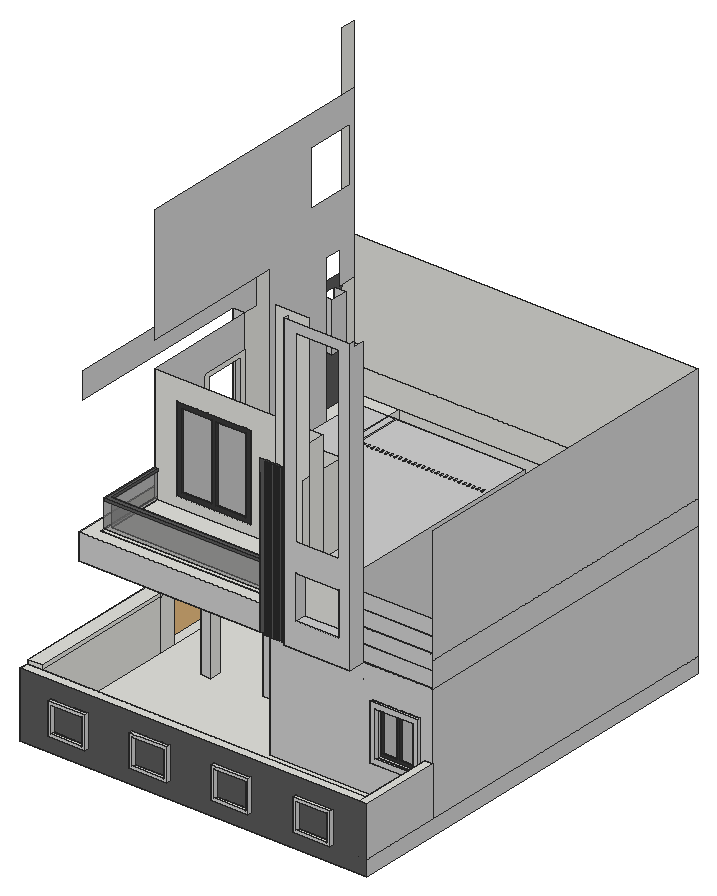
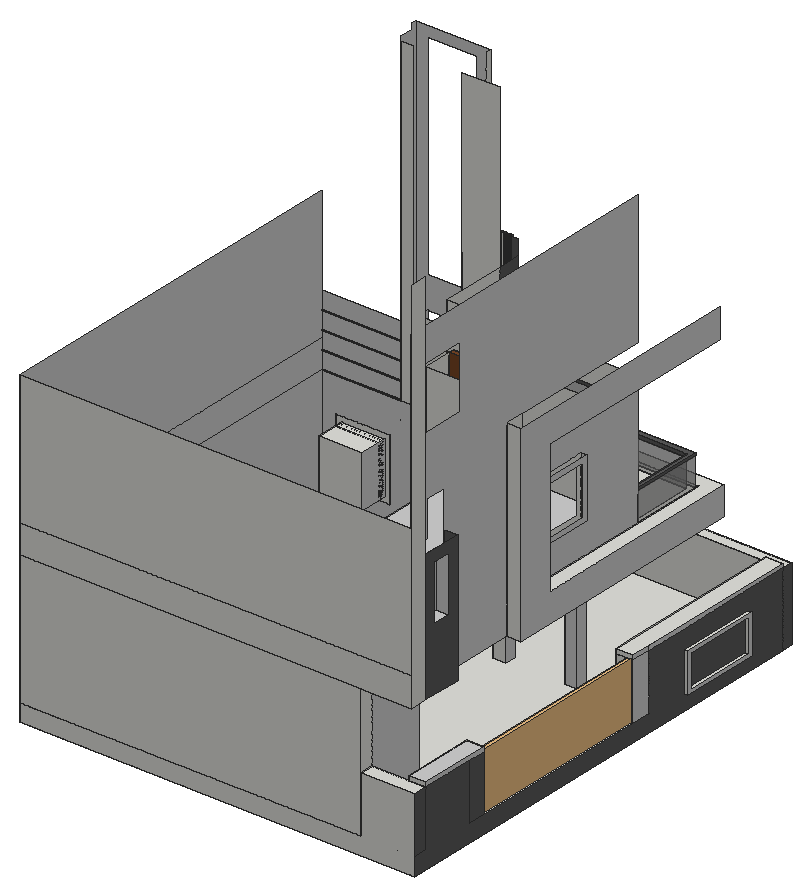
# SketchUp Ruby script. Lengths in inches.
U = 1.inch
M = Sketchup.active_model
def pt(a) = Geom::Point3d.new(a.map { |v| v * U })
def face(e, loops, mat)
  f = e.add_face(loops[0].map { |a| pt(a) })
  loops[1..].each { |l| e.add_face(l.map { |a| pt(a) }).erase! }
  f.material = f.back_material = mat if mat
  f
end
# faces: each face lists its corners as indices into pts; further lists are holes
def faces(e, pts, list, mat = nil) = list.each { |f| face(e, (f[0].is_a?(Array) ? f : [f]).map { |l| l.map { |i| pts[i] } }, mat) }
# xy, xz, yz: faces in a plane at the given z, y or x. An outline is a flat list of corners, or four numbers for a rectangle; further outlines are holes
def ring(l) = l.size == 4 ? [[l[0], l[1]], [l[2], l[1]], [l[2], l[3]], [l[0], l[3]]] : l.each_slice(2).to_a
def flat(e, list, mat, &to3) = list.each { |f| face(e, (f[0].is_a?(Array) ? f : [f]).map { |l| ring(l).map { |u, v| to3.(u, v) } }, mat) }
def xy(e, z, list, mat = nil) = flat(e, list, mat) { |x, y| [x, y, z] }
def xz(e, y, list, mat = nil) = flat(e, list, mat) { |x, z| [x, y, z] }
def yz(e, x, list, mat = nil) = flat(e, list, mat) { |y, z| [x, y, z] }
def lines(e, pts, list) = list.each { |a, b| e.add_line(pt(pts[a]), pt(pts[b])) }
# prism: a flat outline (further loops are holes) pulled along v
def prism(e, loops, v, mat = nil)
  f = face(e, loops, mat); d = Geom::Vector3d.new(v.map { |x| x * U })
  f.pushpull(f.normal.samedirection?(d) ? d.length : -d.length)
end
def box(e, o, s, mat = nil) = prism(e, [[o, [o[0] + s[0], o[1], o[2]], [o[0] + s[0], o[1] + s[1], o[2]], [o[0], o[1] + s[1], o[2]]]], [0, 0, s[2]], mat)
def at(x, y, z, deg = 0) = Geom::Transformation.translation(pt([x, y, z])) * Geom::Transformation.rotation(ORIGIN, Z_AXIS, deg.degrees)
def axes(o, x, y, z) = Geom::Transformation.new([*x, 0, *y, 0, *z, 0, *pt(o).to_a, 1])
def part(name) = M.definitions.add(name)
# library, detail: a bought-in or finely detailed component or shape, given as its bounding box
def library(name, o, s) = part(name).tap { |d| box(d.entities, o, s) }
def detail(e, o, s) = box(e.add_group.entities, o, s)
def put(e, d, t, mat = nil) = e.add_instance(d, t).tap { |i| i.material = mat if mat }
def group(e, t, mat = nil) = e.add_group.tap { |g| g.transformation = t; g.material = mat if mat }.entities
root = M.entities
M.materials.add("Generic").color = [90, 90, 90]
M.materials.add("Generic\#1").color = [208, 208, 208]
M.materials.add("[Color M07]").color = [58, 58, 58]
M.materials.add("[Mirror 01]").color = [185, 185, 185]
M.materials.add("[Translucent Glass Gray]").color = [128, 128, 128]
M.materials["[Translucent Glass Gray]"].alpha = 0.5
M.materials.add("[Wood Bamboo]").color = [177, 105, 43]
M.materials.add("[Wood Veneer 01]").color = [120, 70, 37]
c1 = library("Group\#6",[0,0,0],[5.12,237.75,72])
c2 = part("Group\#5")
xy(c2.entities,225.125,[[0,0,3,3.25]])
xz(c2.entities,0,[[0,0,3,225.125]])
yz(c2.entities,0,[[0,0,3.25,225.125]])
yz(c2.entities,3,[[0,0,3.25,225.125]])
c3 = part("Group\#8")
xy(c3.entities,0,[[0,0,56.875,6.5]],"[Wood Veneer 01]")
xy(c3.entities,4.88,[[4.88,0,51.99,3.5]],"[Wood Veneer 01]")
xy(c3.entities,109.93,[[4.88,0,51.99,3.5]],"[Wood Veneer 01]")
xy(c3.entities,114.8125,[[0,0,56.875,6.5]],"[Wood Veneer 01]")
xz(c3.entities,0,[[[0,0,56.875,114.8125],[4.88,4.88,51.99,109.93]]],"[Wood Veneer 01]")
xz(c3.entities,0.5,[[8.38,56.46,8.6,56.49,8.8,56.57,8.97,56.7,9.1,56.88,9.1875,57.08,9.22,57.3,9.1875,57.51,9.1,57.71,8.97,57.89,8.8,58.02,8.6,58.1,8.38,58.13,8.16,58.1,7.96,58.02,7.79,57.89,7.66,57.71,7.57,57.51,7.54,57.3,7.57,57.08,7.66,56.88,7.79,56.7,7.96,56.57,8.16,56.49]],"[Wood Veneer 01]")
xz(c3.entities,3.5,[[8.38,56.46,8.16,56.49,7.96,56.57,7.79,56.7,7.66,56.88,7.57,57.08,7.54,57.3,7.57,57.51,7.66,57.71,7.79,57.89,7.96,58.02,8.16,58.1,8.38,58.13,8.6,58.1,8.8,58.02,8.97,57.89,9.1,57.71,9.1875,57.51,9.22,57.3,9.1875,57.08,9.1,56.88,8.97,56.7,8.8,56.57,8.6,56.49]])
xz(c3.entities,3.5,[[[4.88,4.88,51.99,109.93],[8.38,56.46,8.16,56.49,7.96,56.57,7.79,56.7,7.66,56.88,7.57,57.08,7.54,57.3,7.57,57.51,7.66,57.71,7.79,57.89,7.96,58.02,8.16,58.1,8.38,58.13,8.6,58.1,8.8,58.02,8.97,57.89,9.1,57.71,9.1875,57.51,9.22,57.3,9.1875,57.08,9.1,56.88,8.97,56.7,8.8,56.57,8.6,56.49]]],"[Wood Bamboo]")
xz(c3.entities,6.5,[[0,0,56.875,114.8125]],"[Wood Veneer 01]")
yz(c3.entities,0,[[0,0,6.5,114.8125]],"[Wood Veneer 01]")
yz(c3.entities,4.88,[[0,4.88,3.5,109.93]],"[Wood Veneer 01]")
yz(c3.entities,51.99,[[0,4.88,3.5,109.93]],"[Wood Veneer 01]")
yz(c3.entities,56.875,[[0,0,6.5,114.8125]],"[Wood Veneer 01]")
p = [[7.96,3.5,56.57],[8.16,3.5,56.49],[8.16,0.5,56.49],[7.96,0.5,56.57],[8.38,3.5,56.46],[8.38,0.5,56.46],
  [8.6,3.5,56.49],[8.6,0.5,56.49],[8.8,3.5,56.57],[8.8,0.5,56.57],[7.79,3.5,56.7],[7.79,0.5,56.7],
  [8.97,3.5,56.7],[8.97,0.5,56.7],[7.66,3.5,56.88],[7.66,0.5,56.88],[9.1,3.5,56.88],[9.1,0.5,56.88],
  [7.57,3.5,57.08],[7.57,0.5,57.08],[9.1875,3.5,57.08],[9.1875,0.5,57.08],[7.54,3.5,57.3],[7.54,0.5,57.3],
  [9.22,3.5,57.3],[9.22,0.5,57.3],[7.57,3.5,57.51],[7.57,0.5,57.51],[9.1875,3.5,57.51],[9.1875,0.5,57.51],
  [7.66,3.5,57.71],[7.66,0.5,57.71],[9.1,3.5,57.71],[9.1,0.5,57.71],[7.79,3.5,57.89],[7.79,0.5,57.89],
  [8.97,3.5,57.89],[8.97,0.5,57.89],[7.96,3.5,58.02],[7.96,0.5,58.02],[8.8,3.5,58.02],[8.8,0.5,58.02],
  [8.16,3.5,58.1],[8.16,0.5,58.1],[8.6,3.5,58.1],[8.6,0.5,58.1],[8.38,3.5,58.13],[8.38,0.5,58.13],
  [8.38,3.5,57.3],[8.38,0.5,57.3]]
faces(c3.entities,p,[[0,1,2,3],[1,4,5,2],[4,6,7,5],[6,8,9,7],[10,0,3,11],[8,12,13,9],[14,10,11,15],[12,16,17,13],
  [18,14,15,19],[16,20,21,17],[22,18,19,23],[20,24,25,21],[26,22,23,27],[24,28,29,25],[30,26,27,31],[28,32,33,29],
  [34,30,31,35],[32,36,37,33],[38,34,35,39],[36,40,41,37],[42,38,39,43],[40,44,45,41],[46,42,43,47],[44,46,47,45]],"[Wood Veneer 01]")
lines(c3.entities,p,[[48,49]])
c4 = part("Group\#7")
xy(c4.entities,0,[[0,0,106.25,6]],"[Color M07]")
xy(c4.entities,6.42,[[6.42,0,49.92,3],[56.33,0,99.83,3]],"[Color M07]")
xy(c4.entities,116.15,[[6.42,0,49.92,3],[56.33,0,99.83,3]],"[Color M07]")
xy(c4.entities,122.5625,[[0,0,106.25,6]],"[Color M07]")
xz(c4.entities,0,[[[0,0,106.25,122.5625],[56.33,6.42,99.83,116.15],[6.42,6.42,49.92,116.15]]],"[Color M07]")
xz(c4.entities,3,[[6.42,6.42,49.92,116.15],[56.33,6.42,99.83,116.15]],"[Mirror 01]")
xz(c4.entities,6,[[0,0,106.25,122.5625]],"[Mirror 01]")
yz(c4.entities,0,[[0,0,6,122.5625]],"[Color M07]")
yz(c4.entities,6.42,[[0,6.42,3,116.15]],"[Color M07]")
yz(c4.entities,49.92,[[0,6.42,3,116.15]],"[Color M07]")
yz(c4.entities,56.33,[[0,6.42,3,116.15]],"[Color M07]")
yz(c4.entities,99.83,[[0,6.42,3,116.15]],"[Color M07]")
yz(c4.entities,106.25,[[0,0,6,122.5625]],"[Color M07]")
xy(root,-21.6875,[[5.4375,5.4375,507.1875,19],[5.4375,19,27.1875,605.125],[27.1875,19,507.1875,605.125]])
xy(root,-1.26,[[0,75.49,5.4375,176.95]],"Generic\#1")
xy(root,0,[[[27.1875,19,495.5625,19,495.5625,125.125,271.1875,125.125,271.1875,512.5,251.64,512.5,251.64,524.5,199.78,524.5,199.78,512.5,73.6875,512.5,73.6875,587,27.1875,587],[180.62,226.81,197.18,241.25],[93.57,221.98,108.82,237.23]],[495.5625,19,507.1875,125.125],[271.1875,125.125,507.1875,125.125,507.1875,605.125,73.6875,605.125,73.6875,587,271.1875,587],[5.4375,233.125,27.1875,257.3125],[5.4375,257.3125,27.1875,495.0625],
  [5.4375,495.0625,27.1875,519.25],[85,524.5,271.1875,587]])
xy(root,0,[[73.6875,512.5,85,587],[85,512.5,199.78,524.5],[251.64,512.5,271.1875,524.5]],"Generic\#1")
xy(root,1.89,[[404.83,0,458.61,5.4375]])
xy(root,1.89,[[49.9,0,103.67,5.4375],[168.21,0,221.98,5.4375],[286.52,0,340.3,5.4375]],"Generic\#1")
xy(root,2.75,[[0,79.5,5.4375,172.9375]])
xy(root,5.91,[[53.91,0,99.66,5.4375],[290.53,0,336.28,5.4375],[408.85,0,454.6,5.4375]])
xy(root,5.91,[[172.22,0,217.97,5.4375]],"Generic\#1")
xy(root,44.09,[[408.85,0,454.6,5.4375]])
xy(root,44.09,[[53.91,0,99.66,5.4375],[172.22,0,217.97,5.4375],[290.53,0,336.28,5.4375]],"Generic\#1")
xy(root,44.88,[[0,79.5,5.4375,172.9375]])
xy(root,45.03,[[420.53,120.5625,489.125,125.125]])
xy(root,48.11,[[404.83,0,458.61,5.4375]])
xy(root,48.11,[[49.9,0,103.67,5.4375],[168.21,0,221.98,5.4375],[286.52,0,340.3,5.4375]],"Generic\#1")
xy(root,48.89,[[0,75.49,5.4375,176.95]])
xy(root,51.86,[[427.36,120.5625,482.3,125.125],[427.36,125.125,482.3,160.875]],"Generic\#1")
xy(root,72,[[5.4375,5.4375,495.5625,19],[495.5625,5.4375,507.1875,125.125],[5.4375,19,27.1875,233.125],[5.4375,233.125,27.1875,257.3125],[5.4375,495.0625,27.1875,519.25],
  [5.4375,519.25,27.1875,587],[5.4375,587,73.6875,605.125]])
xy(root,77.5,[[5.4375,19,27.1875,257.3125]])
xy(root,77.5,[[5.4375,495.0625,27.1875,587]],"Generic\#1")
xy(root,89.9375,[[199.78,512.5,251.64,524.5]],"Generic\#1")
xy(root,117.55,[[427.36,120.5625,482.3,125.125],[427.36,125.125,482.3,160.875]])
xy(root,124.375,[[420.53,120.5625,489.125,125.125]],"Generic\#1")
xy(root,131.75,[[[85,512.5,271.1875,512.5,271.1875,516.95,270.34,516.95,270.34,521.26,271.1875,521.26,271.1875,524.5,85,524.5],[263.71,516.95,265.46,521.26],[257.09,516.95,258.84,521.26],[250.46,516.95,252.21,521.26],[243.84,516.95,245.59,521.26],[237.21,516.95,238.96,521.26],[230.59,516.95,232.34,521.26],[223.96,516.95,225.71,521.26],[217.34,516.95,219.09,521.26],[204.09,516.95,205.84,521.26],[197.46,516.95,199.21,521.26],[190.84,516.95,192.59,521.26],[184.21,516.95,185.96,521.26],[177.59,516.95,179.34,521.26],[170.96,516.95,172.71,521.26],[164.34,516.95,166.09,521.26],[157.71,516.95,159.46,521.26],[151.09,516.95,152.84,521.26],[144.46,516.95,146.21,521.26],[137.84,516.95,139.59,521.26],[131.21,516.95,132.96,521.26],[124.59,516.95,126.34,521.26],[117.96,516.95,119.71,521.26],[111.34,516.95,113.09,521.26],[104.71,516.95,106.46,521.26],[98.09,516.95,99.84,521.26],[91.46,516.95,93.21,521.26],[210.71,516.95,212.46,521.26]],[91.46,516.95,93.21,521.26],[98.09,516.95,99.84,521.26],[104.71,516.95,106.46,521.26],[111.34,516.95,113.09,521.26],
  [117.96,516.95,119.71,521.26],[124.59,516.95,126.34,521.26],[131.21,516.95,132.96,521.26],[137.84,516.95,139.59,521.26],[144.46,516.95,146.21,521.26],
  [151.09,516.95,152.84,521.26],[157.71,516.95,159.46,521.26],[164.34,516.95,166.09,521.26],[170.96,516.95,172.71,521.26],[177.59,516.95,179.34,521.26],
  [184.21,516.95,185.96,521.26],[190.84,516.95,192.59,521.26],[197.46,516.95,199.21,521.26],[204.09,516.95,205.84,521.26],[210.71,516.95,212.46,521.26],
  [217.34,516.95,219.09,521.26],[223.96,516.95,225.71,521.26],[230.59,516.95,232.34,521.26],[237.21,516.95,238.96,521.26],[243.84,516.95,245.59,521.26],
  [250.46,516.95,252.21,521.26],[257.09,516.95,258.84,521.26],[263.71,516.95,265.46,521.26],[270.34,516.95,271.1875,521.26],[271.1875,516.95,272.09,521.26],
  [276.96,516.95,278.71,521.26],[283.59,516.95,285.34,521.26],[290.21,516.95,291.96,521.26],[296.84,516.95,298.59,521.26],[303.46,516.95,305.21,521.26],
  [310.09,516.95,311.84,521.26],[316.71,516.95,318.46,521.26],[323.34,516.95,325.09,521.26],[329.96,516.95,331.71,521.26],[336.59,516.95,338.34,521.26],
  [343.21,516.95,344.96,521.26],[349.84,516.95,351.59,521.26],[356.46,516.95,358.21,521.26],[363.09,516.95,364.84,521.26],[369.71,516.95,371.46,521.26]],"Generic\#1")
xy(root,168,[[311.625,101.1875,328.9375,108.0625],[9.25,531.8125,27.1875,583.375],[9.25,583.375,9.25,605.125,73.6875,605.125,73.6875,587,27.1875,587,27.1875,583.375]])
xy(root,168,[[328.9375,101.1875,328.9375,108.0625,307.5625,108.0625,307.5625,104.8125,304.5625,104.8125,304.5625,108.0625,271.1875,108.0625,271.1875,125.125,406.8125,125.125,406.8125,101.1875],[9.25,108.0625,9.25,430.9,27.1875,430.9,27.1875,125.125,271.1875,125.125,271.1875,108.0625],[[27.1875,125.125,27.1875,587,73.6875,587,73.6875,512.5,85,512.5,85,587,271.1875,587,271.1875,125.125],[180.62,226.81,197.18,241.25],[93.57,221.98,108.82,237.23],[91.46,516.95,93.21,521.26],[98.09,516.95,99.84,521.26],[104.71,516.95,106.46,521.26],[111.34,516.95,113.09,521.26],[117.96,516.95,119.71,521.26],[124.59,516.95,126.34,521.26],[131.21,516.95,132.96,521.26],[137.84,516.95,139.59,521.26],[144.46,516.95,146.21,521.26],[151.09,516.95,152.84,521.26],[157.71,516.95,159.46,521.26],[164.34,516.95,166.09,521.26],[170.96,516.95,172.71,521.26],[263.71,516.95,265.46,521.26],[257.09,516.95,258.84,521.26],[250.46,516.95,252.21,521.26],[243.84,516.95,245.59,521.26],[237.21,516.95,238.96,521.26],[230.59,516.95,232.34,521.26],[223.96,516.95,225.71,521.26],[217.34,516.95,219.09,521.26],[204.09,516.95,205.84,521.26],[177.59,516.95,179.34,521.26],[184.21,516.95,185.96,521.26],[190.84,516.95,192.59,521.26],[197.46,516.95,199.21,521.26],[210.71,516.95,212.46,521.26]],[73.6875,512.5,85,587]],"Generic\#1")
xy(root,169.18,[[406.8125,125.125,507.1875,125.875]])
xy(root,170.18,[[406.8125,125.125,507.1875,125.875]])
xy(root,191.75,[[406.8125,125.125,507.1875,126.125]])
xy(root,192.75,[[406.8125,125.125,507.1875,126.125]])
xy(root,205.3125,[[9.25,108.0625,271.1875,108.0625,271.1875,125.125,27.1875,125.125,27.1875,385.65,9.25,385.65],[27.1875,125.125,271.1875,130.75],[271.1875,125.125,319.1875,137],[27.1875,130.75,27.1875,222.125,32.1875,222.125,32.1875,138,271.1875,138,271.1875,130.75],[32.1875,138,32.1875,222.125,205.46,222.125,205.46,266.625,262.34,266.625,262.34,222.125,271.1875,222.125,271.1875,138]])
xy(root,205.3125,[[328.9375,101.1875,391.1875,116.5]],"Generic\#1")
xy(root,214.32,[[406.8125,125.125,507.1875,126.125]])
xy(root,215.32,[[406.8125,125.125,507.1875,126.125]])
xy(root,219.84,[[59.8,222.125,166.05,244.9375]])
xy(root,236.89,[[406.8125,125.125,507.1875,126.125]])
xy(root,237.89,[[406.8125,125.125,507.1875,126.125]])
xy(root,241.3125,[[27.1875,130.75,27.1875,222.125,32.1875,222.125,32.1875,138,271.1875,138,271.1875,130.75]])
xy(root,245.3125,[[27.1875,130.75,271.1875,130.75,271.1875,138,32.1875,138,32.1875,222.125,27.1875,222.125]],"Generic")
xy(root,248.82,[[9.25,545.63,25.375,569.56]],"Generic\#1")
xy(root,250.2,[[19.75,313.34,27.1875,385.65]],"Generic\#1")
xz(root,0,[[[49.9,1.89,103.67,48.11],[53.91,5.91,99.66,44.09]],[[168.21,1.89,221.98,48.11],[172.22,5.91,217.97,44.09]],[[286.52,1.89,340.3,48.11],[290.53,5.91,336.28,44.09]],[[404.83,1.89,458.61,48.11],[408.85,5.91,454.6,44.09]]],"Generic\#1")
xz(root,5.4375,[[[49.9,1.89,103.67,48.11],[53.91,5.91,99.66,44.09]],[[168.21,1.89,221.98,48.11],[172.22,5.91,217.97,44.09]],[[286.52,1.89,340.3,48.11],[290.53,5.91,336.28,44.09]],[[404.83,1.89,458.61,48.11],[408.85,5.91,454.6,44.09]]])
xz(root,5.4375,[[[5.4375,-21.6875,507.1875,72],[404.83,1.89,458.61,48.11],[49.9,1.89,103.67,48.11],[168.21,1.89,221.98,48.11],[286.52,1.89,340.3,48.11]],[53.91,5.91,99.66,44.09],[172.22,5.91,217.97,44.09],[290.53,5.91,336.28,44.09],[408.85,5.91,454.6,44.09]],"Generic")
xz(root,19,[[5.4375,-21.6875,27.1875,72],[27.1875,0,495.5625,72],[5.4375,72,27.1875,77.5]])
xz(root,75.49,[[0,-1.26,5.4375,48.89]],"Generic\#1")
xz(root,79.5,[[0,2.75,5.4375,44.88]])
xz(root,101.1875,[[[311.625,168,406.8125,591.5625],[328.9375,306.96,391.1875,578.625],[328.9375,205.3125,391.1875,267.4]]],"Generic\#1")
xz(root,108.0625,[[280.1875,168,283.1875,393.125],[285.0625,168,288.0625,393.125],[289.9375,168,292.9375,393.125],[294.8125,168,297.8125,393.125],[299.6875,168,302.6875,393.125]])
xz(root,108.0625,[[271.1875,168,280.1875,393.125],[283.1875,168,285.0625,393.125],[288.0625,168,289.9375,393.125],[292.9375,168,294.8125,393.125],[297.8125,168,299.6875,393.125],
  [302.6875,168,304.5625,393.125],[307.5625,168,311.625,393.125]],"Generic")
xz(root,108.0625,[[9.25,168,271.1875,205.3125]],"Generic\#1")
xz(root,116.5,[[328.9375,205.3125,391.1875,267.4]])
xz(root,120.5625,[[[420.53,45.03,489.125,124.375],[427.36,51.86,482.3,117.55]]],"Generic\#1")
xz(root,125.125,[[495.5625,0,507.1875,72],[[420.53,45.03,489.125,124.375],[427.36,51.86,482.3,117.55]],[27.1875,168,271.1875,205.3125],[271.1875,168,319.1875,205.3125],[391.1875,168,406.8125,578.625]])
xz(root,125.125,[[[271.1875,0,495.5625,0,495.5625,72,507.1875,72,507.1875,169.18,406.8125,169.18,406.8125,168,271.1875,168],[420.53,45.03,489.125,124.375]],[406.8125,170.18,507.1875,191.75],[406.8125,192.75,507.1875,214.32],[406.8125,215.32,507.1875,236.89],[406.8125,237.89,507.1875,259.46]],"Generic\#1")
xz(root,125.875,[[406.8125,169.18,507.1875,170.18]])
xz(root,126.125,[[406.8125,191.75,507.1875,192.75],[406.8125,214.32,507.1875,215.32],[406.8125,236.89,507.1875,237.89]])
xz(root,130.75,[[27.1875,241.3125,271.1875,245.3125]],"Generic")
xz(root,130.75,[[27.1875,205.3125,271.1875,241.3125]],"[Translucent Glass Gray]")
xz(root,137,[[271.1875,205.3125,319.1875,578.625]])
xz(root,138,[[32.1875,241.3125,271.1875,245.3125]],"Generic")
xz(root,138,[[32.1875,205.3125,271.1875,241.3125]],"[Translucent Glass Gray]")
xz(root,160.875,[[427.36,51.86,482.3,117.55]])
xz(root,172.9375,[[0,2.75,5.4375,44.88]],"Generic\#1")
xz(root,176.95,[[0,-1.26,5.4375,48.89]])
xz(root,221.98,[[93.57,0,108.82,168]],"Generic\#1")
xz(root,222.125,[[[32.1875,205.3125,205.46,205.3125,205.46,320.125,262.34,320.125,262.34,205.3125,271.1875,205.3125,271.1875,373.3125,27.1875,373.3125,27.1875,245.3125,32.1875,245.3125],[59.8,219.84,166.05,342.41]]])
xz(root,226.81,[[180.62,0,197.18,168]],"Generic\#1")
xz(root,233.125,[[5.4375,0,27.1875,72]])
xz(root,237.23,[[93.57,0,108.82,168]],"Generic\#1")
xz(root,241.25,[[180.62,0,197.18,168]])
xz(root,244.9375,[[59.8,219.84,166.05,342.41]])
xz(root,257.3125,[[5.4375,0,27.1875,72],[5.4375,72,27.1875,77.5]])
xz(root,266.625,[[205.46,205.3125,262.34,320.125]])
xz(root,313.34,[[19.75,250.2,27.1875,325.58]],"Generic\#1")
xz(root,385.65,[[19.75,250.2,27.1875,325.58]])
xz(root,385.65,[[9.25,205.3125,27.1875,205.3125,27.1875,250.2,19.75,250.2,19.75,325.58,27.1875,325.58,27.1875,373.3125,9.25,373.3125]],"Generic\#1")
xz(root,430.9,[[9.25,168,27.1875,410.625]])
xz(root,495.0625,[[5.4375,0,27.1875,72]],"Generic")
xz(root,495.0625,[[5.4375,72,27.1875,77.5]],"Generic\#1")
xz(root,512.5,[[73.6875,0,85,168],[85,0,199.78,0,199.78,89.9375,251.64,89.9375,251.64,0,271.1875,0,271.1875,131.75,85,131.75]],"Generic\#1")
xz(root,516.95,[[91.46,131.75,93.21,168],[98.09,131.75,99.84,168],[104.71,131.75,106.46,168],[111.34,131.75,113.09,168],[117.96,131.75,119.71,168],
  [124.59,131.75,126.34,168],[131.21,131.75,132.96,168],[137.84,131.75,139.59,168],[144.46,131.75,146.21,168],[151.09,131.75,152.84,168],
  [157.71,131.75,159.46,168],[164.34,131.75,166.09,168],[170.96,131.75,172.71,168],[177.59,131.75,179.34,168],[184.21,131.75,185.96,168],
  [190.84,131.75,192.59,168],[197.46,131.75,199.21,168],[204.09,131.75,205.84,168],[210.71,131.75,212.46,168],[217.34,131.75,219.09,168],
  [223.96,131.75,225.71,168],[230.59,131.75,232.34,168],[237.21,131.75,238.96,168],[243.84,131.75,245.59,168],[250.46,131.75,252.21,168],
  [257.09,131.75,258.84,168],[263.71,131.75,265.46,168]],"Generic\#1")
xz(root,519.25,[[5.4375,0,27.1875,72]])
xz(root,521.26,[[91.46,131.75,93.21,168],[98.09,131.75,99.84,168],[104.71,131.75,106.46,168],[111.34,131.75,113.09,168],[117.96,131.75,119.71,168],
  [124.59,131.75,126.34,168],[131.21,131.75,132.96,168],[137.84,131.75,139.59,168],[144.46,131.75,146.21,168],[151.09,131.75,152.84,168],
  [157.71,131.75,159.46,168],[164.34,131.75,166.09,168],[170.96,131.75,172.71,168],[177.59,131.75,179.34,168],[184.21,131.75,185.96,168],
  [190.84,131.75,192.59,168],[197.46,131.75,199.21,168],[204.09,131.75,205.84,168],[210.71,131.75,212.46,168],[217.34,131.75,219.09,168],
  [223.96,131.75,225.71,168],[230.59,131.75,232.34,168],[237.21,131.75,238.96,168],[243.84,131.75,245.59,168],[250.46,131.75,252.21,168],
  [257.09,131.75,258.84,168],[263.71,131.75,265.46,168]],"Generic\#1")
xz(root,524.5,[[85,0,85,131.75,271.1875,131.75,271.1875,0,251.64,0,251.64,89.9375,199.78,89.9375,199.78,0]],"Generic\#1")
xz(root,531.8125,[[9.25,168,27.1875,333.84]],"Generic")
xz(root,545.63,[[9.25,248.82,25.375,320.02]],"Generic\#1")
xz(root,569.56,[[9.25,248.82,25.375,320.02]],"Generic\#1")
xz(root,587,[[5.4375,0,27.1875,72],[27.1875,0,73.6875,72],[5.4375,72,27.1875,77.5]])
xz(root,587,[[73.6875,0,85,168],[85,0,271.1875,168]],"Generic\#1")
xz(root,605.125,[[5.4375,-21.6875,5.4375,72,73.6875,72,73.6875,0,507.1875,0,507.1875,-21.6875],[73.6875,0,507.1875,168],[9.25,168,507.1875,205.3125],[9.25,205.3125,507.1875,373.3125]])
yz(root,0,[[[75.49,-1.26,176.95,48.89],[79.5,2.75,172.9375,44.88]]],"Generic\#1")
yz(root,5.4375,[[5.4375,-21.6875,19,72],[[19,-21.6875,19,72,233.125,72,233.125,0,519.25,0,519.25,72,587,72,587,0,605.125,0,605.125,-21.6875],[75.49,-1.26,176.95,48.89]],[495.0625,0,519.25,72],[587,0,605.125,72],[79.5,2.75,172.9375,44.88]],"Generic")
yz(root,5.4375,[[233.125,0,257.3125,72],[19,72,233.125,77.5],[233.125,72,257.3125,77.5],[495.0625,72,587,77.5]],"Generic\#1")
yz(root,9.25,[[583.375,168,605.125,650.4375]])
yz(root,9.25,[[[531.8125,168,583.375,333.84],[545.63,248.82,569.56,320.02]]],"Generic")
yz(root,9.25,[[108.0625,168,108.0625,205.3125,385.65,205.3125,385.65,373.3125,115,373.3125,115,410.625,430.9,410.625,430.9,168]],"Generic\#1")
yz(root,19.75,[[[313.34,250.2,385.65,325.58],[319.97,256.83,379.02,318.95]]],"Generic\#1")
yz(root,25.375,[[545.63,248.82,569.56,320.02]],"Generic\#1")
yz(root,27.1875,[[19,0,233.125,72],[233.125,0,257.3125,72],[495.0625,0,519.25,72],[519.25,0,587,72],[19,72,233.125,77.5],
  [233.125,72,257.3125,77.5],[495.0625,72,519.25,77.5],[519.25,72,587,77.5],[125.125,168,430.9,205.3125],[385.65,205.3125,385.65,373.3125,407.53,373.3125,407.53,410.625,430.9,410.625,430.9,205.3125],
  [[313.34,250.2,385.65,325.58],[319.97,256.83,379.02,318.95]]])
yz(root,27.1875,[[130.75,241.3125,222.125,245.3125]],"Generic")
yz(root,27.1875,[[[430.9,168,430.9,410.625,222.125,410.625,222.125,578.625,583.375,578.625,583.375,333.84,557.59,333.84,557.59,380.36,531.8125,380.36,531.8125,168],[505.08,456.26,574.96,535.64]],[222.125,205.3125,222.125,373.3125,385.65,373.3125,385.65,325.58,313.34,325.58,313.34,250.2,385.65,250.2,385.65,205.3125]],"Generic\#1")
yz(root,27.1875,[[130.75,205.3125,222.125,241.3125]],"[Translucent Glass Gray]")
yz(root,32.1875,[[138,241.3125,222.125,245.3125]],"Generic")
yz(root,32.1875,[[138,205.3125,222.125,241.3125]],"[Translucent Glass Gray]")
yz(root,49.9,[[0,1.89,5.4375,48.11]],"Generic\#1")
yz(root,53.91,[[0,5.91,5.4375,44.09]],"Generic\#1")
yz(root,59.8,[[222.125,219.84,244.9375,342.41]])
yz(root,73.6875,[[587,0,605.125,72],[587,72,605.125,168]])
yz(root,73.6875,[[512.5,0,587,168]],"Generic\#1")
yz(root,85,[[512.5,0,524.5,131.75],[524.5,0,587,72],[524.5,72,587,72,587,168,512.5,168,512.5,131.75,524.5,131.75]],"Generic\#1")
yz(root,91.46,[[516.95,131.75,521.26,168]],"Generic\#1")
yz(root,93.21,[[516.95,131.75,521.26,168]],"Generic\#1")
yz(root,93.57,[[221.98,0,237.23,168]],"Generic\#1")
yz(root,98.09,[[516.95,131.75,521.26,168]],"Generic\#1")
yz(root,99.66,[[0,5.91,5.4375,44.09]],"Generic\#1")
yz(root,99.84,[[516.95,131.75,521.26,168]],"Generic\#1")
yz(root,103.67,[[0,1.89,5.4375,48.11]],"Generic\#1")
yz(root,104.71,[[516.95,131.75,521.26,168]],"Generic\#1")
yz(root,106.46,[[516.95,131.75,521.26,168]],"Generic\#1")
yz(root,108.82,[[221.98,0,237.23,168]])
yz(root,111.34,[[516.95,131.75,521.26,168]],"Generic\#1")
yz(root,113.09,[[516.95,131.75,521.26,168]],"Generic\#1")
yz(root,117.96,[[516.95,131.75,521.26,168]],"Generic\#1")
yz(root,119.71,[[516.95,131.75,521.26,168]],"Generic\#1")
yz(root,124.59,[[516.95,131.75,521.26,168]],"Generic\#1")
yz(root,126.34,[[516.95,131.75,521.26,168]],"Generic\#1")
yz(root,131.21,[[516.95,131.75,521.26,168]],"Generic\#1")
yz(root,132.96,[[516.95,131.75,521.26,168]],"Generic\#1")
yz(root,137.84,[[516.95,131.75,521.26,168]],"Generic\#1")
yz(root,139.59,[[516.95,131.75,521.26,168]],"Generic\#1")
yz(root,144.46,[[516.95,131.75,521.26,168]],"Generic\#1")
yz(root,146.21,[[516.95,131.75,521.26,168]],"Generic\#1")
yz(root,151.09,[[516.95,131.75,521.26,168]],"Generic\#1")
yz(root,152.84,[[516.95,131.75,521.26,168]],"Generic\#1")
yz(root,157.71,[[516.95,131.75,521.26,168]],"Generic\#1")
yz(root,159.46,[[516.95,131.75,521.26,168]],"Generic\#1")
yz(root,164.34,[[516.95,131.75,521.26,168]],"Generic\#1")
yz(root,166.05,[[222.125,219.84,244.9375,342.41]])
yz(root,166.09,[[516.95,131.75,521.26,168]],"Generic\#1")
yz(root,168.21,[[0,1.89,5.4375,48.11]],"Generic\#1")
yz(root,170.96,[[516.95,131.75,521.26,168]],"Generic\#1")
yz(root,172.22,[[0,5.91,5.4375,44.09]],"Generic\#1")
yz(root,172.71,[[516.95,131.75,521.26,168]],"Generic\#1")
yz(root,177.59,[[516.95,131.75,521.26,168]],"Generic\#1")
yz(root,179.34,[[516.95,131.75,521.26,168]],"Generic\#1")
yz(root,180.62,[[226.81,0,241.25,168]],"Generic\#1")
yz(root,184.21,[[516.95,131.75,521.26,168]],"Generic\#1")
yz(root,185.96,[[516.95,131.75,521.26,168]],"Generic\#1")
yz(root,190.84,[[516.95,131.75,521.26,168]],"Generic\#1")
yz(root,192.59,[[516.95,131.75,521.26,168]],"Generic\#1")
yz(root,197.18,[[226.81,0,241.25,168]])
yz(root,197.46,[[516.95,131.75,521.26,168]],"Generic\#1")
yz(root,199.21,[[516.95,131.75,521.26,168]],"Generic\#1")
yz(root,199.78,[[512.5,0,524.5,89.9375]],"Generic\#1")
yz(root,204.09,[[516.95,131.75,521.26,168]],"Generic\#1")
yz(root,205.46,[[222.125,205.3125,266.625,320.125]])
yz(root,205.84,[[516.95,131.75,521.26,168]],"Generic\#1")
yz(root,210.71,[[516.95,131.75,521.26,168]],"Generic\#1")
yz(root,212.46,[[516.95,131.75,521.26,168]],"Generic\#1")
yz(root,217.34,[[516.95,131.75,521.26,168]],"Generic\#1")
yz(root,217.97,[[0,5.91,5.4375,44.09]],"Generic\#1")
yz(root,219.09,[[516.95,131.75,521.26,168]],"Generic\#1")
yz(root,221.98,[[0,1.89,5.4375,48.11]],"Generic\#1")
yz(root,223.96,[[516.95,131.75,521.26,168]],"Generic\#1")
yz(root,225.71,[[516.95,131.75,521.26,168]],"Generic\#1")
yz(root,230.59,[[516.95,131.75,521.26,168]],"Generic\#1")
yz(root,232.34,[[516.95,131.75,521.26,168]],"Generic\#1")
yz(root,237.21,[[516.95,131.75,521.26,168]],"Generic\#1")
yz(root,238.96,[[516.95,131.75,521.26,168]],"Generic\#1")
yz(root,243.84,[[516.95,131.75,521.26,168]],"Generic\#1")
yz(root,245.59,[[516.95,131.75,521.26,168]],"Generic\#1")
yz(root,250.46,[[516.95,131.75,521.26,168]],"Generic\#1")
yz(root,251.64,[[512.5,0,524.5,89.9375]],"Generic\#1")
yz(root,252.21,[[516.95,131.75,521.26,168]],"Generic\#1")
yz(root,257.09,[[516.95,131.75,521.26,168]],"Generic\#1")
yz(root,258.84,[[516.95,131.75,521.26,168]],"Generic\#1")
yz(root,262.34,[[222.125,205.3125,266.625,320.125]])
yz(root,263.71,[[516.95,131.75,521.26,168]],"Generic\#1")
yz(root,265.46,[[516.95,131.75,521.26,168]],"Generic\#1")
yz(root,271.1875,[[108.0625,168,125.125,205.3125],[130.75,205.3125,137,241.3125],[137,205.3125,138,241.3125],[138,205.3125,138,245.3125,137,245.3125,137,373.3125,222.125,373.3125,222.125,205.3125],[130.75,241.3125,137,245.3125],
  [137,241.3125,138,245.3125]])
yz(root,271.1875,[[108.0625,205.3125,108.0625,373.3125,137,373.3125,137,245.3125,130.75,245.3125,130.75,205.3125]],"Generic")
yz(root,271.1875,[[125.125,0,125.125,168,587,168,587,0,524.5,0,524.5,131.75,512.5,131.75,512.5,0]],"Generic\#1")
yz(root,286.52,[[0,1.89,5.4375,48.11]],"Generic\#1")
yz(root,290.53,[[0,5.91,5.4375,44.09]],"Generic\#1")
yz(root,311.625,[[101.1875,168,101.1875,591.5625,108.0625,591.5625,108.0625,573.5,109.1875,573.5,109.1875,572.5,108.0625,572.5,108.0625,560.6875,109.1875,560.6875,109.1875,559.6875,108.0625,559.6875,108.0625,547.875,109.1875,547.875,109.1875,546.875,108.0625,546.875,108.0625,535.0625,109.1875,535.0625,109.1875,534.0625,108.0625,534.0625,108.0625,522.25,109.1875,522.25,109.1875,521.25,108.0625,521.25,108.0625,509.4375,109.1875,509.4375,109.1875,508.4375,108.0625,508.4375,108.0625,496.625,109.1875,496.625,109.1875,495.625,108.0625,495.625,108.0625,483.8125,109.1875,483.8125,109.1875,482.8125,108.0625,482.8125,108.0625,471,109.1875,471,109.1875,470,108.0625,470,108.0625,458.1875,109.1875,458.1875,109.1875,457.1875,108.0625,457.1875,108.0625,445.375,109.1875,445.375,109.1875,444.375,108.0625,444.375,108.0625,432.5625,109.1875,432.5625,109.1875,431.5625,108.0625,431.5625,108.0625,419.75,109.1875,419.75,109.1875,418.75,108.0625,418.75,108.0625,406.9375,109.1875,406.9375,109.1875,405.9375,108.0625,405.9375,108.0625,394.125,109.1875,394.125,109.1875,393.125,108.0625,393.125,108.0625,168]])
yz(root,319.1875,[[125.125,205.3125,137,373.3125]])
yz(root,328.9375,[[101.1875,205.3125,116.5,267.4]],"Generic\#1")
yz(root,336.28,[[0,5.91,5.4375,44.09]])
yz(root,340.3,[[0,1.89,5.4375,48.11]],"Generic\#1")
yz(root,391.1875,[[116.5,205.3125,125.125,267.4]])
yz(root,391.1875,[[101.1875,205.3125,116.5,267.4]],"Generic\#1")
yz(root,404.83,[[0,1.89,5.4375,48.11]],"Generic\#1")
yz(root,406.8125,[[125.125,169.18,125.875,170.18],[125.125,191.75,126.125,192.75],[125.125,214.32,126.125,215.32],[125.125,236.89,126.125,237.89]])
yz(root,406.8125,[[101.1875,168,125.125,168,125.125,584.3125,108.0625,584.3125,108.0625,591.5625,101.1875,591.5625]],"Generic\#1")
yz(root,408.85,[[0,5.91,5.4375,44.09]],"Generic\#1")
yz(root,420.53,[[120.5625,45.03,125.125,124.375]])
yz(root,427.36,[[120.5625,51.86,125.125,117.55],[125.125,51.86,160.875,117.55]],"Generic\#1")
yz(root,454.6,[[0,5.91,5.4375,44.09]])
yz(root,458.61,[[0,1.89,5.4375,48.11]],"Generic\#1")
yz(root,482.3,[[120.5625,51.86,125.125,117.55],[125.125,51.86,160.875,117.55]],"Generic\#1")
yz(root,489.125,[[120.5625,45.03,125.125,124.375]],"Generic\#1")
yz(root,495.5625,[[19,0,125.125,72]])
yz(root,507.1875,[[5.4375,-21.6875,605.125,0],[5.4375,0,125.125,72],[125.125,0,605.125,168],[125.125,168,605.125,168,605.125,205.3125,125.125,205.3125,125.125,192.75,126.125,192.75,126.125,191.75,125.125,191.75,125.125,170.18,125.875,170.18,125.875,169.18,125.125,169.18],[125.125,205.3125,605.125,205.3125,605.125,373.3125,126.125,373.3125,126.125,372.3125,125.125,372.3125,125.125,350.74,126.125,350.74,126.125,349.74,125.125,349.74,125.125,328.17,126.125,328.17,126.125,327.17,125.125,327.17,125.125,305.6,126.125,305.6,126.125,304.6,125.125,304.6,125.125,283.03,126.125,283.03,126.125,282.03,125.125,282.03,125.125,260.46,126.125,260.46,126.125,259.46,125.125,259.46,125.125,237.89,126.125,237.89,126.125,236.89,125.125,236.89,125.125,215.32,126.125,215.32,126.125,214.32,125.125,214.32]],"Generic\#1")
p = [[27.1875,605.125,0],[27.1875,587,0],[406.8125,125.125,146.61],[406.8125,125.125,147.61],[495.5625,19,0],[495.5625,5.4375,0]]
lines(root,p,[[0,1],[2,3],[4,5]])
put(root,c1,at(8.32,257.3125,0))
g1 = group(root,at(427.36,128.75,51.86))
xy(g1,0,[[0,0,54.9375,6]],"[Color M07]")
xy(g1,4.14,[[4.14,0,25.4,3],[29.54,0,50.8,3]],"[Color M07]")
xy(g1,61.55,[[4.14,0,25.4,3],[29.54,0,50.8,3]],"[Color M07]")
xy(g1,65.6875,[[0,0,54.9375,6]],"[Color M07]")
xz(g1,0,[[[0,0,54.9375,65.6875],[4.14,4.14,25.4,61.55],[29.54,4.14,50.8,61.55]]],"[Color M07]")
xz(g1,3,[[4.14,4.14,25.4,61.55],[29.54,4.14,50.8,61.55]],"[Mirror 01]")
xz(g1,6,[[0,0,54.9375,65.6875]],"[Mirror 01]")
yz(g1,0,[[0,0,6,65.6875]],"[Color M07]")
yz(g1,4.14,[[0,4.14,3,61.55]],"[Color M07]")
yz(g1,25.4,[[0,4.14,3,61.55]],"[Color M07]")
yz(g1,29.54,[[0,4.14,3,61.55]],"[Color M07]")
yz(g1,50.8,[[0,4.14,3,61.55]],"[Color M07]")
yz(g1,54.9375,[[0,0,6,65.6875]],"[Color M07]")
put(root,c2,at(304.5625,104.8125,168),"Generic")
put(root,c2,at(299.6875,104.8125,168),"Generic")
put(root,c2,at(294.8125,104.8125,168),"Generic")
put(root,c2,at(289.9375,104.8125,168),"Generic")
put(root,c2,at(285.0625,104.8125,168),"Generic")
put(root,c2,at(280.1875,104.8125,168),"Generic")
put(root,c3,at(205.46,222.125,205.3125))
put(root,c4,at(59.8,222.125,219.84))
